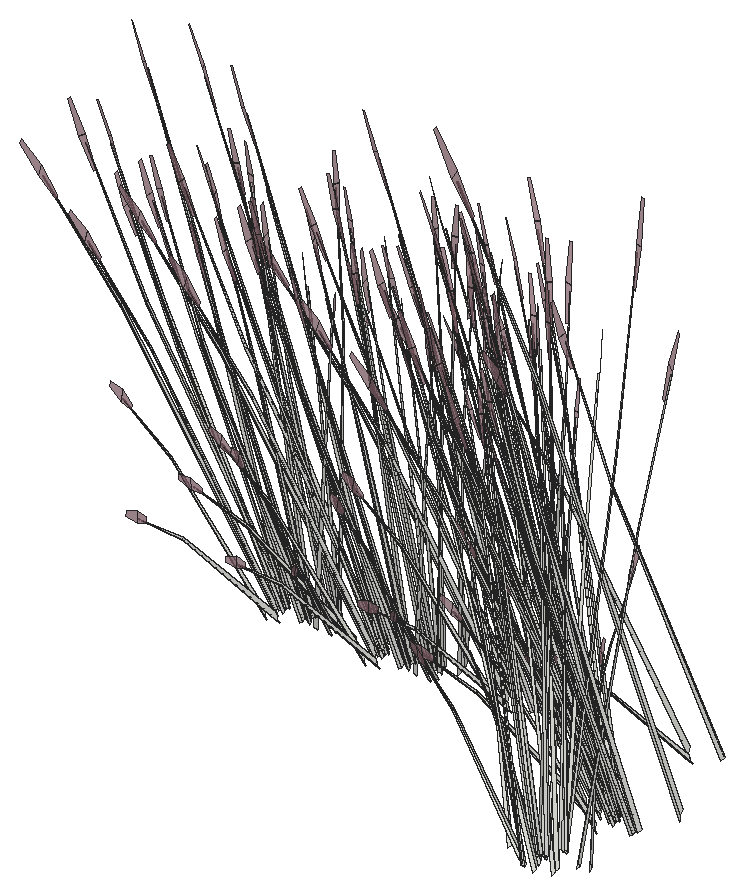
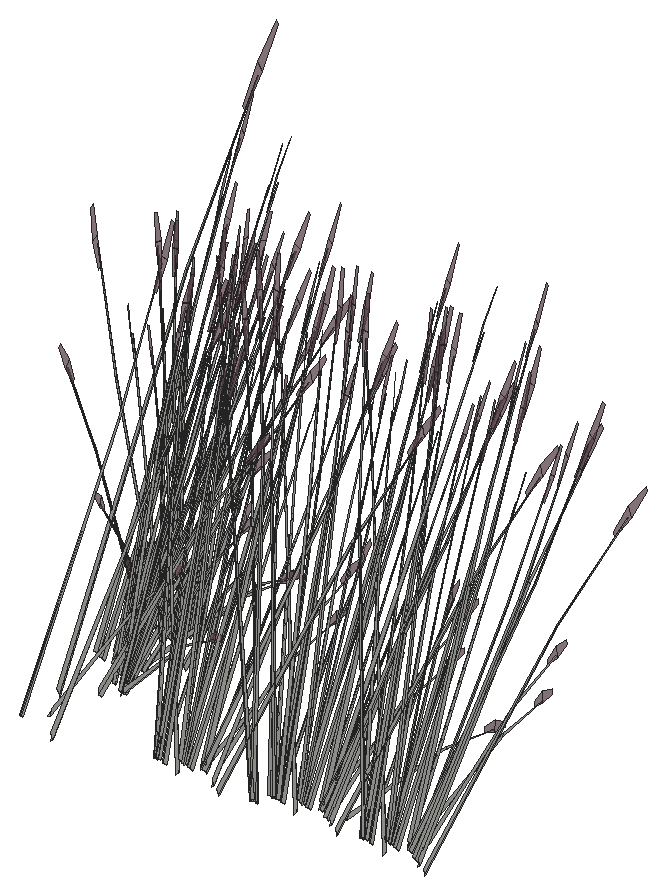
# SketchUp Ruby script. Lengths in inches.
U = 1.inch
M = Sketchup.active_model
def pt(a) = Geom::Point3d.new(a.map { |v| v * U })
def face(e, loops, mat)
  f = e.add_face(loops[0].map { |a| pt(a) })
  loops[1..].each { |l| e.add_face(l.map { |a| pt(a) }).erase! }
  f.material = f.back_material = mat if mat
  f
end
# faces: each face lists its corners as indices into pts; further lists are holes
def faces(e, pts, list, mat = nil) = list.each { |f| face(e, (f[0].is_a?(Array) ? f : [f]).map { |l| l.map { |i| pts[i] } }, mat) }
# xy, xz, yz: faces in a plane at the given z, y or x. An outline is a flat list of corners, or four numbers for a rectangle; further outlines are holes
def ring(l) = l.size == 4 ? [[l[0], l[1]], [l[2], l[1]], [l[2], l[3]], [l[0], l[3]]] : l.each_slice(2).to_a
def flat(e, list, mat, &to3) = list.each { |f| face(e, (f[0].is_a?(Array) ? f : [f]).map { |l| ring(l).map { |u, v| to3.(u, v) } }, mat) }
def xy(e, z, list, mat = nil) = flat(e, list, mat) { |x, y| [x, y, z] }
def xz(e, y, list, mat = nil) = flat(e, list, mat) { |x, z| [x, y, z] }
def yz(e, x, list, mat = nil) = flat(e, list, mat) { |y, z| [x, y, z] }
def lines(e, pts, list) = list.each { |a, b| e.add_line(pt(pts[a]), pt(pts[b])) }
# prism: a flat outline (further loops are holes) pulled along v
def prism(e, loops, v, mat = nil)
  f = face(e, loops, mat); d = Geom::Vector3d.new(v.map { |x| x * U })
  f.pushpull(f.normal.samedirection?(d) ? d.length : -d.length)
end
def box(e, o, s, mat = nil) = prism(e, [[o, [o[0] + s[0], o[1], o[2]], [o[0] + s[0], o[1] + s[1], o[2]], [o[0], o[1] + s[1], o[2]]]], [0, 0, s[2]], mat)
def at(x, y, z, deg = 0) = Geom::Transformation.translation(pt([x, y, z])) * Geom::Transformation.rotation(ORIGIN, Z_AXIS, deg.degrees)
def axes(o, x, y, z) = Geom::Transformation.new([*x, 0, *y, 0, *z, 0, *pt(o).to_a, 1])
def part(name) = M.definitions.add(name)
# library, detail: a bought-in or finely detailed component or shape, given as its bounding box
def library(name, o, s) = part(name).tap { |d| box(d.entities, o, s) }
def detail(e, o, s) = box(e.add_group.entities, o, s)
def put(e, d, t, mat = nil) = e.add_instance(d, t).tap { |i| i.material = mat if mat }
def group(e, t, mat = nil) = e.add_group.tap { |g| g.transformation = t; g.material = mat if mat }.entities
root = M.entities
M.materials.add("LightPink_Translucent").color = [144, 107, 117]
M.materials["LightPink_Translucent"].alpha = 0.75
c1 = part("blade")
p = [[2.15,0.21,22],[0,0.17,0],[0.09,0.45,0],[2.18,0.31,22],[2.29,0.31,22],[0.38,0.45,0],
  [2.48,0.24,33],[2.49,0.24,33],[2.48,0.22,33]]
faces(c1.entities,p,[[0,1,2,3],[4,5,2,3],[6,3,4,7],[8,0,3,6]])
c2 = part("seeds")
p = [[0.3,-0.1,1.38],[-0.01,-0.03,1.59],[-0.01,-0.03,0.03],[0.14,-0.07,-0.07],[0.29,-0.03,3],[0.15,0.01,3.11]]
faces(c2.entities,p,[[0,1,2,3],[1,0,4,5]],"LightPink_Translucent")
c3 = part("blade with seeds")
put(c3.entities,c1,at(0,0,0))
put(c3.entities,c2,axes([2.4,0.25,30.99],[1.5799,-0.05474,1.17369],[-0.12525,1.92788,0.29478],[-0.07173,-0.02425,1.56792]))
put(root,c3,axes([684.11,322.09,267.91],[-0.10624,0.07413,1.45204],[0.00904,0.54162,-0.22964],[-0.24352,0.07044,0.11645]))
put(root,c3,axes([684.82,322.01,267.89],[-0.17625,0.51936,-0.42412],[-0.60429,-0.17802,-0.32852],[-0.2433,0.04762,0.81151]))
put(root,c3,axes([684.8,321.57,268.18],[0.32734,0.51701,-0.10093],[-0.58097,0.25407,-0.56021],[-0.24483,0.06821,0.85122]))
put(root,c3,axes([686.74,328.07,267.89],[-0.63954,-0.14313,-0.42412],[0.21921,-0.49074,-0.32852],[-0.05864,-0.19758,0.81151]))
put(root,c3,axes([685.6,326.55,267.91],[-0.01214,0.06844,1.47228],[-0.59861,0.24837,-0.13912],[-0.17615,-0.12696,0.26054]))
put(root,c3,axes([684.72,323.02,267.93],[-0.16135,-0.52549,0.39842],[0.63294,-0.0912,0.32852],[-0.18654,0.12359,0.82444]))
put(root,c3,axes([684.6,322.91,267.93],[-0.44663,-0.24013,0.05337],[0.26003,-0.34195,0.42015],[-0.14319,0.11055,0.64067]))
put(root,c3,axes([684.8,322.28,267.22],[0.22574,-0.12077,1.42242],[0.19004,0.55807,0.11501],[-0.35439,0.12613,0.60807]))
put(root,c3,axes([685.46,327.76,268.23],[0.72473,-0.14676,0.44623],[0.12578,0.57568,0.36794],[-0.17045,-0.16967,0.92337]))
put(root,c3,axes([687.29,328.04,268.18],[-0.63664,0.26583,-0.10093],[-0.31286,-0.47181,-0.56021],[-0.084,-0.19882,0.85122]))
put(root,c3,axes([685.57,328.29,268.13],[-0.55475,-0.27598,-0.58968],[0.39425,-0.48361,0.07116],[-0.20099,-0.16478,0.83415]))
put(root,c3,axes([685.38,327.93,267.76],[-0.10048,-0.4599,-0.29394],[0.5744,-0.12144,0.37948],[-0.15428,-0.13179,0.72609]))
put(root,c3,axes([685.11,322.84,268.19],[0.56631,-0.0816,0.29394],[0.14954,0.46647,-0.37948],[-0.16229,0.12529,0.72609]))
put(root,c3,axes([682.93,322.63,267.91],[0.08303,0.01531,1.47228],[0.25685,0.50448,-0.13912],[-0.16996,0.13241,0.26054]))
put(root,c3,axes([683.63,324.24,266.3],[0.27113,-0.25877,0.95334],[0.10699,0.40966,0.70045],[-0.19594,0.07335,0.20998]))
put(root,c3,axes([685.63,327.89,267.93],[0.29569,-0.36271,0.05337],[0.42107,0.21117,0.42015],[-0.13613,-0.11629,0.64067]))
put(root,c3,axes([684.65,323.12,267.76],[-0.56631,0.0816,-0.29394],[-0.14954,-0.46647,0.37948],[-0.16229,0.12529,0.72609]))
put(root,c3,axes([684.15,328.6,267.22],[0.24166,0.09837,1.42242],[-0.50011,0.41269,0.11501],[-0.3117,-0.18617,0.60807]))
put(root,c3,axes([685.31,328.31,267.89],[-0.64198,0.13573,-0.42412],[-0.1123,-0.514,-0.32852],[-0.17243,-0.1473,0.81151]))
put(root,c3,axes([685.76,327.85,268.51],[-0.4342,0.54737,-0.11304],[-0.6288,-0.31535,-0.62743],[-0.21858,-0.15465,0.95337]))
put(root,c3,axes([683.83,324.17,268.6875],[0.5741,0.15241,-0.05385],[-0.1766,0.46909,-0.24415],[-0.0939,0.07122,0.8053]))
put(root,c3,axes([684.82,322.8,268.18],[0.60181,0.31483,-0.10093],[-0.34671,0.45593,-0.56021],[-0.17003,0.15849,0.85122]))
put(root,c3,axes([684.1,327.69,267.91],[-0.13998,-0.00403,1.45204],[-0.44565,0.40302,-0.22964],[-0.23779,-0.08235,0.11645]))
put(root,c3,axes([685.63,322.66,267.22],[0.1625,-0.17544,1.42242],[0.41029,0.47354,0.11501],[-0.28141,0.21565,0.60807]))
put(root,c3,axes([685.12,323.17,267.89],[0.16713,0.52135,-0.42412],[-0.63294,0.0912,-0.32852],[-0.18138,0.14003,0.81151]))
put(root,c3,axes([686.9,331.41,266.76],[0.56221,0.23024,1.25546],[-0.55078,0.49601,0.49647],[-0.2467,-0.29398,1.05249]))
put(root,c3,axes([685.72,328.3,268.19],[0.10048,0.4599,0.29394],[-0.5744,0.12144,-0.37948],[-0.15428,-0.13179,0.72609]))
put(root,c3,axes([684,328.6,268.23],[0.53728,-0.42137,0.44623],[0.46337,0.44748,0.36794],[-0.25207,-0.07773,0.92337]))
put(root,c3,axes([685.48,324.04,267.93],[-0.53464,-0.0266,0.05337],[0.01466,-0.40172,0.42015],[-0.05594,0.15388,0.64067]))
put(root,c3,axes([685.65,324.08,267.93],[-0.46327,-0.38957,0.39842],[0.49199,-0.33598,0.32852],[-0.08546,0.18277,0.82444]))
put(root,c3,axes([684.24,328.6,267.93],[0.03276,-0.43418,0.05337],[0.49468,0.0119,0.42015],[-0.18949,-0.04543,0.64067]))
put(root,c3,axes([684.05,328.74,267.76],[-0.37017,-0.35748,-0.29394],[0.42268,-0.3384,0.37948],[-0.21476,-0.05149,0.72609]))
put(root,c3,axes([685.51,323.09,267.22],[0.12114,-0.19625,1.42242],[0.50818,0.40613,0.11501],[-0.22925,0.25313,0.60807]))
put(root,c3,axes([685.65,324.2,267.76],[-0.4402,0.30062,-0.29394],[-0.41671,-0.34326,0.37948],[-0.0634,0.1744,0.72609]))
put(root,c3,axes([684.13,324.11,267.91],[-0.01617,0.11299,1.45204],[0.45894,0.39307,-0.22964],[-0.12015,0.18588,0.11645]))
put(root,c3,axes([684.44,328.97,268.13],[-0.65035,-0.01375,-0.58968],[0.04368,-0.5789,0.07116],[-0.27552,-0.06109,0.83415]))
put(root,c3,axes([685.93,325.36,266.3],[-0.01684,-0.3395,0.95334],[0.42072,0.24214,0.70045],[-0.08274,0.16182,0.20998]))
put(root,c3,axes([683.5625,328.03,267.91],[0.04823,0.05698,1.47228],[-0.23252,0.51221,-0.13912],[-0.23548,0.00371,0.26054]))
put(root,c3,axes([684.23,329.09,267.89],[-0.47241,0.37822,-0.42412],[-0.41372,-0.39954,-0.32852],[-0.24002,-0.05755,0.81151]))
put(root,c3,axes([684.58,328.92,268.19],[0.37017,0.35748,0.29394],[-0.42268,0.3384,-0.37948],[-0.21476,-0.05149,0.72609]))
put(root,c3,axes([685.94,323.88,268.43],[-0.01693,0.52814,-0.65454],[-0.71285,-0.03547,0.07899],[-0.07523,0.22375,0.92591]))
put(root,c3,axes([684.08,325.27,267.91],[0.07381,-0.03447,1.47228],[0.61004,0.22929,-0.13912],[-0.01434,0.19091,0.26054]))
put(root,c3,axes([684.48,328.7,268.18],[-0.03484,0.58066,-0.10093],[-0.65957,-0.01587,-0.56021],[-0.25402,-0.04034,0.85122]))
put(root,c3,axes([683.64,329.5,267.22],[0.26985,-0.01293,1.42242],[-0.17902,0.56047,0.11501],[-0.38456,-0.03467,0.60807]))
put(root,c3,axes([665.68,334.09,267.22],[0.14872,0.18332,1.42242],[-0.6872,0.15433,0.11501],[-0.15531,-0.28779,0.60807]))
put(root,c3,axes([666.81,332.875,267.91],[-0.09951,-0.08005,1.45204],[-0.66407,0.05075,-0.22964],[-0.10598,-0.19148,0.11645]))
put(root,c3,axes([667.51,334.23,268.13],[-0.31051,-0.46426,-0.58968],[0.63919,-0.25873,0.07116],[-0.07261,-0.22432,0.83415]))
put(root,c3,axes([658.97,334.625,267.22],[0.14872,0.18332,1.42242],[-0.6872,0.15433,0.11501],[-0.15531,-0.28779,0.60807]))
put(root,c3,axes([673.58,334.68,267.22],[0.14872,0.18332,1.42242],[-0.6872,0.15433,0.11501],[-0.15531,-0.28779,0.60807]))
put(root,c3,axes([683.52,329.92,267.93],[0.18381,-0.5206,0.39842],[0.60429,0.17802,0.32852],[-0.23764,0.03129,0.82444]))
put(root,c3,axes([660.11,333.41,267.91],[-0.09951,-0.08005,1.45204],[-0.66407,0.05075,-0.22964],[-0.10598,-0.19148,0.11645]))
put(root,c3,axes([683.48,329.78,267.93],[-0.23895,-0.38931,0.05337],[0.43573,-0.19055,0.42015],[-0.19208,0.0376,0.64067]))
put(root,c3,axes([668.8,334.68,268.13],[0.01693,-0.52814,-0.58968],[0.71285,0.03547,0.07116],[0.07523,-0.22375,0.83415]))
put(root,c3,axes([674.71,333.47,267.91],[-0.09951,-0.08005,1.45204],[-0.66407,0.05075,-0.22964],[-0.10598,-0.19148,0.11645]))
put(root,c3,axes([685.7,324.62,266.79],[0.01429,-0.29475,1.28107],[0.64291,0.15569,0.17703],[-0.0557,0.31414,0.60492]))
put(root,c3,axes([660.8,334.76,268.13],[-0.31051,-0.46426,-0.58968],[0.63919,-0.25873,0.07116],[-0.07261,-0.22432,0.83415]))
put(root,c3,axes([669.79,333.86,267.91],[-0.00628,-0.11364,1.45204],[-0.53042,-0.32843,-0.22964],[0.08201,-0.19909,0.11645]))
put(root,c3,axes([667.57,333.83,267.76],[0.19614,-0.43908,-0.29394],[0.57222,0.12807,0.37948],[-0.05247,-0.17678,0.72609]))
put(root,c3,axes([668,334.41,267.22],[-0.12114,0.19625,1.42242],[-0.50818,-0.40613,0.11501],[0.22925,-0.25313,0.60807]))
put(root,c3,axes([669.65,333.45,267.91],[-0.06607,0.04361,1.47228],[-0.64734,-0.14714,-0.13912],[-0.02343,-0.19032,0.26054]))
put(root,c3,axes([675.41,334.82,268.13],[-0.31051,-0.46426,-0.58968],[0.63919,-0.25873,0.07116],[-0.07261,-0.22432,0.83415]))
put(root,c3,axes([667.27,334.13,267.89],[-0.63954,-0.14313,-0.42412],[0.21921,-0.49074,-0.32852],[-0.05864,-0.19758,0.81151]))
put(root,c3,axes([668.66,334.5,267.89],[-0.46573,-0.38364,-0.42412],[0.49199,-0.33598,-0.32852],[0.07086,-0.19492,0.81151]))
put(root,c3,axes([662.09,335.22,268.13],[0.01693,-0.52814,-0.58968],[0.71285,0.03547,0.07116],[0.07523,-0.22375,0.83415]))
put(root,c3,axes([683.4,329.98,267.76],[-0.54068,-0.15928,-0.29394],[0.1577,-0.46469,0.37948],[-0.21769,0.04261,0.72609]))
put(root,c3,axes([666.13,332.61,267.91],[-0.01214,0.06844,1.47228],[-0.59861,0.24837,-0.13912],[-0.17615,-0.12696,0.26054]))
put(root,c3,axes([676.7,335.27,268.13],[0.01693,-0.52814,-0.58968],[0.71285,0.03547,0.07116],[0.07523,-0.22375,0.83415]))
put(root,c3,axes([663.09,334.39,267.91],[-0.00628,-0.11364,1.45204],[-0.53042,-0.32843,-0.22964],[0.08201,-0.19909,0.11645]))
put(root,c3,axes([660.86,334.37,267.76],[0.19614,-0.43908,-0.29394],[0.57222,0.12807,0.37948],[-0.05247,-0.17678,0.72609]))
put(root,c3,axes([661.29,334.95,267.22],[-0.12114,0.19625,1.42242],[-0.50818,-0.40613,0.11501],[0.22925,-0.25313,0.60807]))
put(root,c3,axes([662.95,333.98,267.91],[-0.06607,0.04361,1.47228],[-0.64734,-0.14714,-0.13912],[-0.02343,-0.19032,0.26054]))
put(root,c3,axes([677.69,334.45,267.91],[-0.00628,-0.11364,1.45204],[-0.53042,-0.32843,-0.22964],[0.08201,-0.19909,0.11645]))
put(root,c3,axes([675.47,334.43,267.76],[0.19614,-0.43908,-0.29394],[0.57222,0.12807,0.37948],[-0.05247,-0.17678,0.72609]))
put(root,c3,axes([675.9,335.01,267.22],[-0.12114,0.19625,1.42242],[-0.50818,-0.40613,0.11501],[0.22925,-0.25313,0.60807]))
put(root,c3,axes([677.55,334.04,267.91],[-0.06607,0.04361,1.47228],[-0.64734,-0.14714,-0.13912],[-0.02343,-0.19032,0.26054]))
put(root,c3,axes([666,333.83,268.23],[0.72473,-0.14676,0.44623],[0.12578,0.57568,0.36794],[-0.17045,-0.16967,0.92337]))
put(root,c3,axes([667.64,333.93,267.93],[0.64106,0.14927,0.39842],[-0.21921,0.49074,0.32852],[-0.03852,-0.19299,0.82444]))
put(root,c3,axes([660.57,334.67,267.89],[-0.63954,-0.14313,-0.42412],[0.21921,-0.49074,-0.32852],[-0.05864,-0.19758,0.81151]))
put(root,c3,axes([667.82,334.11,268.18],[-0.63664,0.26583,-0.10093],[-0.31286,-0.47181,-0.56021],[-0.084,-0.19882,0.85122]))
put(root,c3,axes([669.14,334.71,268.18],[-0.71502,-0.02829,-0.10093],[0.01954,-0.53563,-0.56021],[0.04967,-0.20629,0.85122]))
put(root,c3,axes([669.09,334.36,267.76],[0.4402,-0.30062,-0.29394],[0.41671,0.34326,0.37948],[0.0634,-0.1744,0.72609]))
put(root,c3,axes([675.17,334.73,267.89],[-0.63954,-0.14313,-0.42412],[0.21921,-0.49074,-0.32852],[-0.05864,-0.19758,0.81151]))
put(root,c3,axes([667.81,333.9,267.93],[0.47939,-0.19405,0.05337],[0.23464,0.35385,0.42015],[-0.0463,-0.15598,0.64067]))
put(root,c3,axes([666.11,334.36,268.13],[-0.55475,-0.27598,-0.58968],[0.39425,-0.48361,0.07116],[-0.20099,-0.16478,0.83415]))
put(root,c3,axes([661.95,335.04,267.89],[-0.46573,-0.38364,-0.42412],[0.49199,-0.33598,-0.32852],[0.07086,-0.19492,0.81151]))
put(root,c3,axes([665.92,333.99,267.76],[-0.10048,-0.4599,-0.29394],[0.5744,-0.12144,0.37948],[-0.15428,-0.13179,0.72609]))
put(root,c3,axes([676.56,335.1,267.89],[-0.46573,-0.38364,-0.42412],[0.49199,-0.33598,-0.32852],[0.07086,-0.19492,0.81151]))
put(root,c3,axes([659.42,333.15,267.91],[-0.01214,0.06844,1.47228],[-0.59861,0.24837,-0.13912],[-0.17615,-0.12696,0.26054]))
put(root,c3,axes([683.97,329.93,268.19],[0.54068,0.15928,0.29394],[-0.1577,0.46469,-0.37948],[-0.21769,0.04261,0.72609]))
put(root,c3,axes([674.03,333.21,267.91],[-0.01214,0.06844,1.47228],[-0.59861,0.24837,-0.13912],[-0.17615,-0.12696,0.26054]))
put(root,c3,axes([659.29,334.36,268.23],[0.72473,-0.14676,0.44623],[0.12578,0.57568,0.36794],[-0.17045,-0.16967,0.92337]))
put(root,c3,axes([673.9,334.42,268.23],[0.72473,-0.14676,0.44623],[0.12578,0.57568,0.36794],[-0.17045,-0.16967,0.92337]))
put(root,c3,axes([685.05,329.9,266.77],[0.18493,-0.0826,1.46963],[0.06377,0.5767,0.11501],[-0.40056,0.07652,0.52526]))
put(root,c3,axes([660.93,334.47,267.93],[0.64106,0.14927,0.39842],[-0.21921,0.49074,0.32852],[-0.03852,-0.19299,0.82444]))
put(root,c3,axes([683.8,336.21,267.22],[0.14872,0.18332,1.42242],[-0.6872,0.15433,0.11501],[-0.15531,-0.28779,0.60807]))
put(root,c3,axes([661.12,334.64,268.18],[-0.63664,0.26583,-0.10093],[-0.31286,-0.47181,-0.56021],[-0.084,-0.19882,0.85122]))
put(root,c3,axes([675.54,334.53,267.93],[0.64106,0.14927,0.39842],[-0.21921,0.49074,0.32852],[-0.03852,-0.19299,0.82444]))
put(root,c3,axes([662.4375,335.24,268.18],[-0.71502,-0.02829,-0.10093],[0.01954,-0.53563,-0.56021],[0.04967,-0.20629,0.85122]))
put(root,c3,axes([666.16,333.95,267.93],[0.29569,-0.36271,0.05337],[0.42107,0.21117,0.42015],[-0.13613,-0.11629,0.64067]))
put(root,c3,axes([662.39,334.9,267.76],[0.4402,-0.30062,-0.29394],[0.41671,0.34326,0.37948],[0.0634,-0.1744,0.72609]))
put(root,c3,axes([675.72,334.7,268.18],[-0.63664,0.26583,-0.10093],[-0.31286,-0.47181,-0.56021],[-0.084,-0.19882,0.85122]))
put(root,c3,axes([661.1,334.43,267.93],[0.47939,-0.19405,0.05337],[0.23464,0.35385,0.42015],[-0.0463,-0.15598,0.64067]))
put(root,c3,axes([659.4,334.89,268.13],[-0.55475,-0.27598,-0.58968],[0.39425,-0.48361,0.07116],[-0.20099,-0.16478,0.83415]))
put(root,c3,axes([677.04,335.3,268.18],[-0.71502,-0.02829,-0.10093],[0.01954,-0.53563,-0.56021],[0.04967,-0.20629,0.85122]))
put(root,c3,axes([684.9375,335,267.91],[-0.09951,-0.08005,1.45204],[-0.66407,0.05075,-0.22964],[-0.10598,-0.19148,0.11645]))
put(root,c3,axes([676.99,334.96,267.76],[0.4402,-0.30062,-0.29394],[0.41671,0.34326,0.37948],[0.0634,-0.1744,0.72609]))
put(root,c3,axes([659.21,334.53,267.76],[-0.10048,-0.4599,-0.29394],[0.5744,-0.12144,0.37948],[-0.15428,-0.13179,0.72609]))
put(root,c3,axes([675.71,334.49,267.93],[0.47939,-0.19405,0.05337],[0.23464,0.35385,0.42015],[-0.0463,-0.15598,0.64067]))
put(root,c3,axes([674.01,334.95,268.13],[-0.55475,-0.27598,-0.58968],[0.39425,-0.48361,0.07116],[-0.20099,-0.16478,0.83415]))
put(root,c3,axes([673.82,334.59,267.76],[-0.10048,-0.4599,-0.29394],[0.5744,-0.12144,0.37948],[-0.15428,-0.13179,0.72609]))
put(root,c3,axes([664.68,334.66,267.22],[0.24166,0.09837,1.42242],[-0.50011,0.41269,0.11501],[-0.3117,-0.18617,0.60807]))
put(root,c3,axes([685.63,336.35,268.13],[-0.31051,-0.46426,-0.58968],[0.63919,-0.25873,0.07116],[-0.07261,-0.22432,0.83415]))
put(root,c3,axes([667.63,334.29,268.19],[-0.19614,0.43908,0.29394],[-0.57222,-0.12807,-0.37948],[-0.05247,-0.17678,0.72609]))
put(root,c3,axes([683.06,330.29,267.91],[-0.10624,0.07413,1.45204],[0.00904,0.54162,-0.22964],[-0.24352,0.07044,0.11645]))
put(root,c3,axes([683.77,330.21,267.89],[-0.17625,0.51936,-0.42412],[-0.60429,-0.17802,-0.32852],[-0.2433,0.04762,0.81151]))
put(root,c3,axes([665.85,334.37,267.89],[-0.64198,0.13573,-0.42412],[-0.1123,-0.514,-0.32852],[-0.17243,-0.1473,0.81151]))
put(root,c3,axes([669.09,334.48,267.93],[0.46327,0.38957,0.39842],[-0.49199,0.33598,0.32852],[0.08546,-0.18277,0.82444]))
put(root,c3,axes([683.74,329.77,268.18],[0.32734,0.51701,-0.10093],[-0.58097,0.25407,-0.56021],[-0.24483,0.06821,0.85122]))
put(root,c3,axes([666.3,333.91,268.51],[-0.4342,0.54737,-0.11304],[-0.6288,-0.31535,-0.62743],[-0.21858,-0.15465,0.95337]))
put(root,c3,axes([669.26,334.52,267.93],[0.53464,0.0266,0.05337],[-0.01466,0.40172,0.42015],[0.05594,-0.15388,0.64067]))
put(root,c3,axes([659.46,334.49,267.93],[0.29569,-0.36271,0.05337],[0.42107,0.21117,0.42015],[-0.13613,-0.11629,0.64067]))
put(root,c3,axes([674.0625,334.55,267.93],[0.29569,-0.36271,0.05337],[0.42107,0.21117,0.42015],[-0.13613,-0.11629,0.64067]))
put(root,c3,axes([668.86,334.79,268.19],[-0.4402,0.30062,0.29394],[-0.41671,-0.34326,-0.37948],[0.0634,-0.1744,0.72609]))
put(root,c3,axes([657.98,335.2,267.22],[0.24166,0.09837,1.42242],[-0.50011,0.41269,0.11501],[-0.3117,-0.18617,0.60807]))
put(root,c3,axes([669.64,335.6,268.13],[0.33983,-0.45051,-0.58968],[0.59551,0.32017,0.07116],[0.20291,-0.16322,0.83415]))
put(root,c3,axes([669.62,335.39,267.89],[-0.16713,-0.52135,-0.42412],[0.63294,-0.0912,-0.32852],[0.18138,-0.14003,0.81151]))
put(root,c3,axes([672.58,335.26,267.22],[0.24166,0.09837,1.42242],[-0.50011,0.41269,0.11501],[-0.3117,-0.18617,0.60807]))
put(root,c3,axes([660.92,334.83,268.19],[-0.19614,0.43908,0.29394],[-0.57222,-0.12807,-0.37948],[-0.05247,-0.17678,0.72609]))
put(root,c3,axes([675.53,334.89,268.19],[-0.19614,0.43908,0.29394],[-0.57222,-0.12807,-0.37948],[-0.05247,-0.17678,0.72609]))
put(root,c3,axes([659.14,334.91,267.89],[-0.64198,0.13573,-0.42412],[-0.1123,-0.514,-0.32852],[-0.17243,-0.1473,0.81151]))
put(root,c3,axes([662.39,335.01,267.93],[0.46327,0.38957,0.39842],[-0.49199,0.33598,0.32852],[0.08546,-0.18277,0.82444]))
put(root,c3,axes([664.63,333.76,267.91],[-0.13998,-0.00403,1.45204],[-0.44565,0.40302,-0.22964],[-0.23779,-0.08235,0.11645]))
put(root,c3,axes([669.92,335.76,268.18],[-0.60181,-0.31483,-0.10093],[0.34671,-0.45593,-0.56021],[0.17003,-0.15849,0.85122]))
